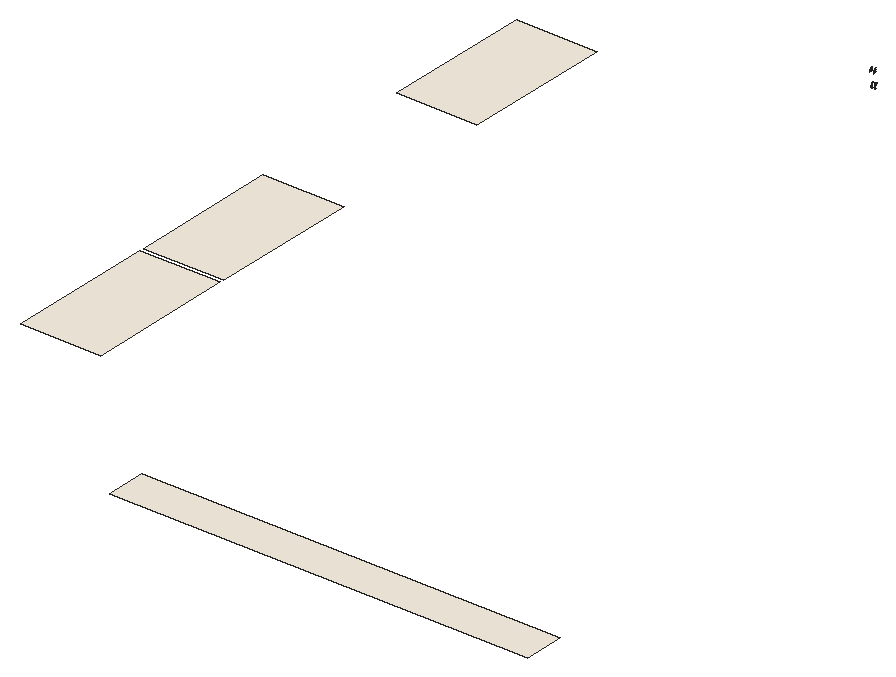
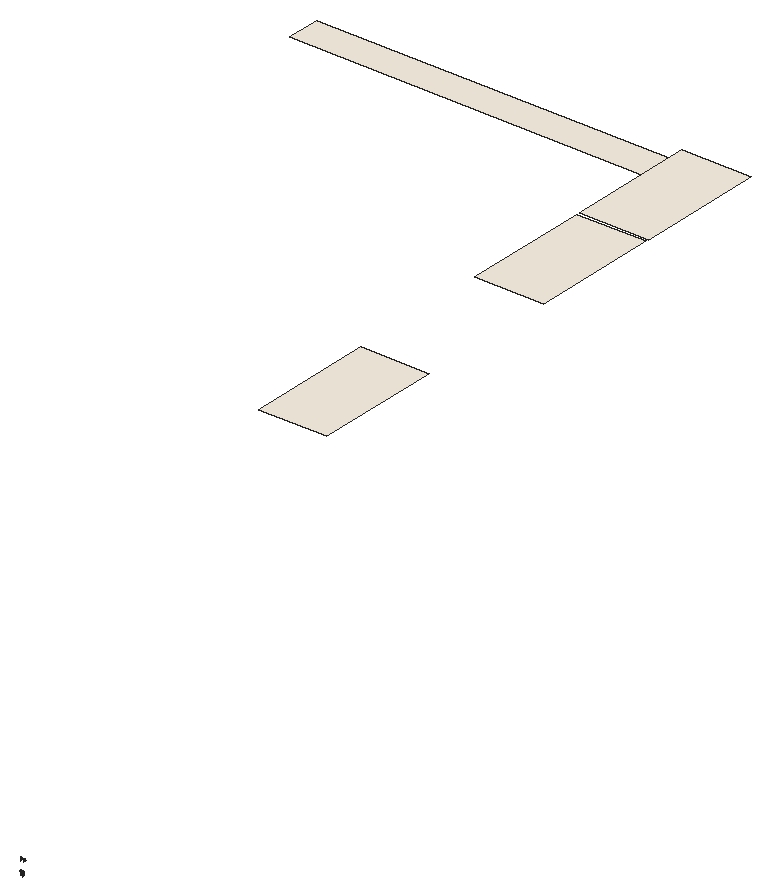
# SketchUp Ruby script. Lengths in inches.
U = 1.inch
M = Sketchup.active_model
def pt(a) = Geom::Point3d.new(a.map { |v| v * U })
def face(e, loops, mat)
  f = e.add_face(loops[0].map { |a| pt(a) })
  loops[1..].each { |l| e.add_face(l.map { |a| pt(a) }).erase! }
  f.material = f.back_material = mat if mat
  f
end
# faces: each face lists its corners as indices into pts; further lists are holes
def faces(e, pts, list, mat = nil) = list.each { |f| face(e, (f[0].is_a?(Array) ? f : [f]).map { |l| l.map { |i| pts[i] } }, mat) }
# xy, xz, yz: faces in a plane at the given z, y or x. An outline is a flat list of corners, or four numbers for a rectangle; further outlines are holes
def ring(l) = l.size == 4 ? [[l[0], l[1]], [l[2], l[1]], [l[2], l[3]], [l[0], l[3]]] : l.each_slice(2).to_a
def flat(e, list, mat, &to3) = list.each { |f| face(e, (f[0].is_a?(Array) ? f : [f]).map { |l| ring(l).map { |u, v| to3.(u, v) } }, mat) }
def xy(e, z, list, mat = nil) = flat(e, list, mat) { |x, y| [x, y, z] }
def xz(e, y, list, mat = nil) = flat(e, list, mat) { |x, z| [x, y, z] }
def yz(e, x, list, mat = nil) = flat(e, list, mat) { |y, z| [x, y, z] }
def lines(e, pts, list) = list.each { |a, b| e.add_line(pt(pts[a]), pt(pts[b])) }
# prism: a flat outline (further loops are holes) pulled along v
def prism(e, loops, v, mat = nil)
  f = face(e, loops, mat); d = Geom::Vector3d.new(v.map { |x| x * U })
  f.pushpull(f.normal.samedirection?(d) ? d.length : -d.length)
end
def box(e, o, s, mat = nil) = prism(e, [[o, [o[0] + s[0], o[1], o[2]], [o[0] + s[0], o[1] + s[1], o[2]], [o[0], o[1] + s[1], o[2]]]], [0, 0, s[2]], mat)
def at(x, y, z, deg = 0) = Geom::Transformation.translation(pt([x, y, z])) * Geom::Transformation.rotation(ORIGIN, Z_AXIS, deg.degrees)
def axes(o, x, y, z) = Geom::Transformation.new([*x, 0, *y, 0, *z, 0, *pt(o).to_a, 1])
def part(name) = M.definitions.add(name)
# library, detail: a bought-in or finely detailed component or shape, given as its bounding box
def library(name, o, s) = part(name).tap { |d| box(d.entities, o, s) }
def detail(e, o, s) = box(e.add_group.entities, o, s)
def put(e, d, t, mat = nil) = e.add_instance(d, t).tap { |i| i.material = mat if mat }
def group(e, t, mat = nil) = e.add_group.tap { |g| g.transformation = t; g.material = mat if mat }.entities
root = M.entities
M.materials.add("Material \#1").color = [140, 140, 140]
M.materials.add("[0030_OldLace]").color = [253, 245, 230]
xy(root,101.375,[[300.251,4.465,393.622,13.465]],"[0030_OldLace]")
xy(root,116.408,[[267,20.993,284.9375,54.346],[267.031,55.388,284.969,88.741],[267.031,126.111,284.969,159.465]],"[0030_OldLace]")
yz(root,265.627,[[260.403,58.146,260.355,58.186,260.316,58.238],[260.416,58.182,260.316,58.238,260.374,58.217],[260.374,58.217,260.316,58.238,260.339,58.263],[260.316,58.238,260.296,58.381,260.3125,58.318],[260.316,58.238,260.3125,58.318,260.339,58.263],
  [260.267,58.371,260.26,58.449,260.262,58.493],[260.262,58.493,260.268,58.536,260.279,58.577],[260.262,58.493,260.626,59.235,260.339,58.634]],"Material \#1")
yz(root,265.641,[[259.87,61.414,259.859,61.415,259.881,61.574],[259.859,61.415,259.87,61.576,259.881,61.574],[260.405,61.519,260.374,61.547,260.382,61.559],[260.405,61.519,260.382,61.559,260.41,61.532],[260.374,61.547,260.348,61.582,260.357,61.591],
  [260.374,61.547,260.357,61.591,260.382,61.559],[259.881,61.574,259.87,61.576,259.911,61.717],[259.87,61.576,259.9,61.723,259.911,61.717],[260.348,61.582,260.327,61.622,260.336,61.63],[260.348,61.582,260.336,61.63,260.357,61.591],
  [260.327,61.622,260.311,61.667,260.321,61.672],[260.327,61.622,260.321,61.672,260.336,61.63],[260.311,61.667,260.3,61.716,260.311,61.718],[260.311,61.667,260.311,61.718,260.321,61.672],[260.3,61.716,260.297,61.772,260.308,61.772],
  [260.3,61.716,260.308,61.772,260.311,61.718],[259.911,61.717,259.9,61.723,259.962,61.857],[259.9,61.723,259.952,61.865,259.962,61.857],[260.297,61.772,260.3,61.819,260.311,61.816],[260.297,61.772,260.311,61.816,260.308,61.772],
  [260.311,61.816,260.3,61.819,260.321,61.862],[260.3,61.819,260.311,61.868,260.321,61.862],[259.962,61.857,259.952,61.865,260.022,61.969],[260.321,61.862,260.311,61.868,260.336,61.905],[259.952,61.865,260.013,61.979,260.022,61.969],
  [260.311,61.868,260.327,61.913,260.336,61.905],[260.336,61.905,260.327,61.913,260.357,61.943],[260.327,61.913,260.348,61.953,260.357,61.943],[260.357,61.943,260.348,61.953,260.382,61.976],[260.348,61.953,260.374,61.987,260.382,61.976],
  [260.022,61.969,260.013,61.979,260.1,62.072],[260.382,61.976,260.374,61.987,260.41,62.003],[260.013,61.979,260.092,62.083,260.1,62.072],[260.374,61.987,260.405,62.016,260.41,62.003],[260.1,62.072,260.092,62.083,260.19,62.156],
  [260.092,62.083,260.184,62.169,260.19,62.156],[260.19,62.156,260.184,62.169,260.29,62.219],[260.184,62.169,260.286,62.233,260.29,62.219],[260.29,62.219,260.286,62.233,260.399,62.258],[260.286,62.233,260.397,62.273,260.399,62.258]],"Material \#1")
yz(root,265.769,[[260.515,58.112,260.316,58.238,260.403,58.146],[260.403,58.146,260.316,58.238,260.355,58.186],[260.416,58.182,260.374,58.217,260.316,58.238],[260.374,58.217,260.339,58.263,260.316,58.238],[260.316,58.238,260.262,58.493,260.267,58.371],
  [260.316,58.238,260.3125,58.318,260.262,58.493],[260.316,58.238,260.267,58.371,260.286,58.301],[260.316,58.238,260.339,58.263,260.3125,58.318],[260.3125,58.318,260.296,58.381,260.262,58.493],[260.267,58.371,260.262,58.493,260.26,58.449],
  [260.296,58.381,260.29,58.449,260.262,58.493],[260.29,58.449,260.296,58.517,260.262,58.493],[260.262,58.493,260.279,58.577,260.268,58.536],[260.262,58.493,260.296,58.517,260.3125,58.579],[260.262,58.493,260.311,58.65,260.279,58.577],
  [260.262,58.493,260.3125,58.579,260.367,58.728],[260.262,58.493,260.36,58.716,260.311,58.65],[260.262,58.493,260.364,58.722,260.36,58.716],[260.262,58.493,260.367,58.728,260.364,58.722],[260.279,58.577,260.311,58.65,260.293,58.615],
  [260.3125,58.579,260.339,58.634,260.367,58.728],[260.311,58.65,260.355,58.71,260.331,58.682],[260.311,58.65,260.36,58.716,260.355,58.71],[260.372,58.757,260.376,59.16,260.372,59.117],[260.376,59.16,260.404,59.235,260.387,59.2],
  [260.376,59.16,260.452,59.286,260.404,59.235]],"Material \#1")
yz(root,266.338,[[260.403,58.146,260.355,58.186,260.316,58.238],[260.416,58.182,260.316,58.238,260.374,58.217],[260.374,58.217,260.316,58.238,260.339,58.263],[260.316,58.238,260.262,58.493,260.3125,58.318],[260.316,58.238,260.267,58.371,260.262,58.493],
  [260.316,58.238,260.286,58.301,260.267,58.371],[260.316,58.238,260.3125,58.318,260.339,58.263],[260.3125,58.318,260.262,58.493,260.296,58.381],[260.267,58.371,260.26,58.449,260.262,58.493],[260.296,58.381,260.262,58.493,260.29,58.449],
  [260.29,58.449,260.262,58.493,260.296,58.517],[260.262,58.493,260.269,58.536,260.279,58.577],[260.262,58.493,260.279,58.577,260.311,58.65],[260.262,58.493,260.311,58.65,260.36,58.716],[260.262,58.493,260.3125,58.579,260.296,58.517],
  [260.262,58.493,260.36,58.716,260.364,58.722],[260.262,58.493,260.364,58.722,260.367,58.728],[260.262,58.493,260.367,58.728,260.3125,58.579],[260.279,58.577,260.293,58.615,260.311,58.65],[260.3125,58.579,260.367,58.728,260.339,58.634],
  [260.311,58.65,260.331,58.682,260.355,58.71],[260.311,58.65,260.355,58.71,260.36,58.716],[260.372,58.757,260.372,59.117,260.376,59.16],[260.372,58.757,260.376,59.16,260.452,59.286],[260.376,59.16,260.387,59.2,260.404,59.235],
  [260.376,59.16,260.404,59.235,260.452,59.286],[260.404,59.235,260.426,59.264,260.452,59.286]],"Material \#1")
yz(root,266.465,[[259.87,61.414,259.881,61.574,259.859,61.415],[259.859,61.415,259.881,61.574,259.87,61.576],[260.405,61.519,260.382,61.559,260.374,61.547],[260.405,61.519,260.41,61.532,260.382,61.559],[260.374,61.547,260.357,61.591,260.348,61.582],
  [260.374,61.547,260.382,61.559,260.357,61.591],[259.881,61.574,259.911,61.717,259.87,61.576],[259.87,61.576,259.911,61.717,259.9,61.723],[260.348,61.582,260.336,61.63,260.327,61.622],[260.348,61.582,260.357,61.591,260.336,61.63],
  [260.327,61.622,260.321,61.672,260.311,61.667],[260.327,61.622,260.336,61.63,260.321,61.672],[260.311,61.667,260.312,61.718,260.3,61.716],[260.311,61.667,260.321,61.672,260.312,61.718],[260.3,61.716,260.308,61.772,260.297,61.772],
  [260.3,61.716,260.312,61.718,260.308,61.772],[259.911,61.717,259.962,61.857,259.9,61.723],[259.9,61.723,259.962,61.857,259.952,61.865],[260.297,61.772,260.308,61.772,260.312,61.816],[260.297,61.772,260.312,61.816,260.3,61.819],
  [260.312,61.816,260.321,61.862,260.3,61.819],[260.3,61.819,260.321,61.862,260.311,61.868],[259.962,61.857,260.022,61.969,259.952,61.865],[260.321,61.862,260.336,61.905,260.311,61.868],[259.952,61.865,260.022,61.969,260.013,61.979],
  [260.311,61.868,260.336,61.905,260.327,61.913],[260.336,61.905,260.357,61.943,260.327,61.913],[260.327,61.913,260.357,61.943,260.348,61.953],[260.357,61.943,260.382,61.976,260.348,61.953],[260.348,61.953,260.382,61.976,260.374,61.987],
  [260.022,61.969,260.1,62.072,260.013,61.979],[260.382,61.976,260.41,62.003,260.374,61.987],[260.013,61.979,260.1,62.072,260.092,62.083],[260.374,61.987,260.41,62.003,260.405,62.016],[260.1,62.072,260.19,62.156,260.092,62.083],
  [260.092,62.083,260.19,62.156,260.184,62.169],[260.19,62.156,260.29,62.219,260.184,62.169],[260.184,62.169,260.29,62.219,260.286,62.233],[260.29,62.219,260.399,62.258,260.286,62.233],[260.286,62.233,260.399,62.258,260.397,62.273]],"Material \#1")
yz(root,266.48,[[260.403,58.146,260.316,58.238,260.355,58.186],[260.416,58.182,260.374,58.217,260.316,58.238],[260.374,58.217,260.339,58.263,260.316,58.238],[260.316,58.238,260.262,58.493,260.267,58.371],[260.316,58.238,260.296,58.381,260.262,58.493],
  [260.316,58.238,260.267,58.371,260.286,58.301],[260.316,58.238,260.3125,58.318,260.296,58.381],[260.316,58.238,260.339,58.263,260.3125,58.318],[260.267,58.371,260.262,58.493,260.26,58.449],[260.296,58.381,260.29,58.449,260.262,58.493],
  [260.29,58.449,260.296,58.517,260.262,58.493],[260.262,58.493,260.279,58.577,260.269,58.536],[260.262,58.493,260.296,58.517,260.3125,58.579],[260.262,58.493,260.311,58.65,260.279,58.577],[260.262,58.493,260.3125,58.579,260.339,58.634],
  [260.262,58.493,260.339,58.634,260.626,59.235],[260.262,58.493,260.36,58.716,260.311,58.65],[260.262,58.493,260.364,58.722,260.36,58.716],[260.262,58.493,260.367,58.728,260.364,58.722],[260.279,58.577,260.311,58.65,260.293,58.615],
  [260.311,58.65,260.355,58.71,260.331,58.682],[260.311,58.65,260.36,58.716,260.355,58.71],[260.372,58.75,260.404,59.235,260.372,58.757],[260.372,58.757,260.376,59.16,260.372,59.117],[260.372,58.757,260.404,59.235,260.376,59.16],
  [260.376,59.16,260.404,59.235,260.387,59.2]],"Material \#1")
